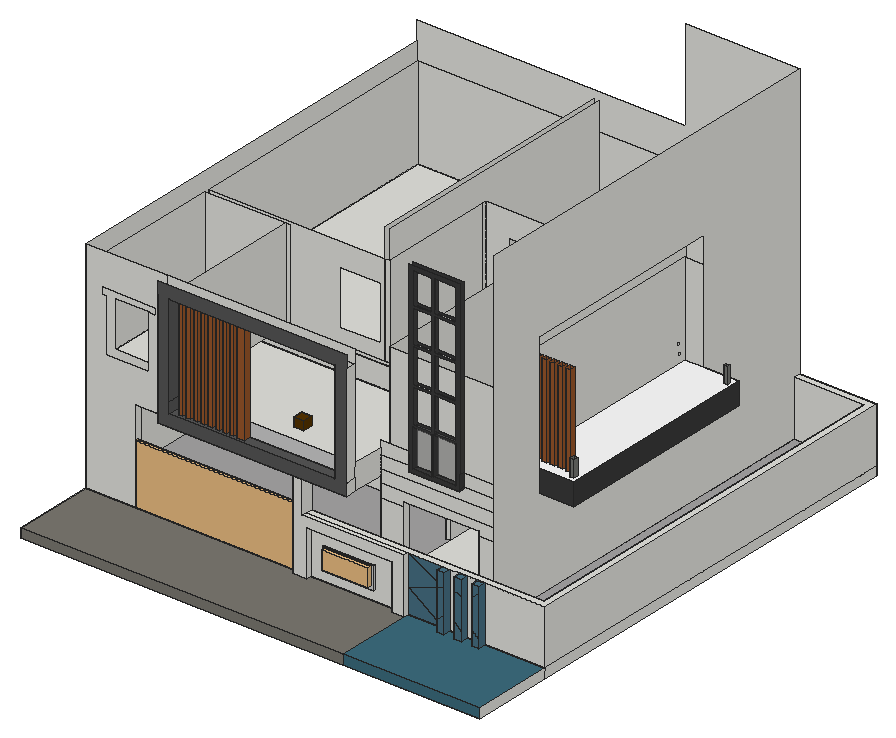
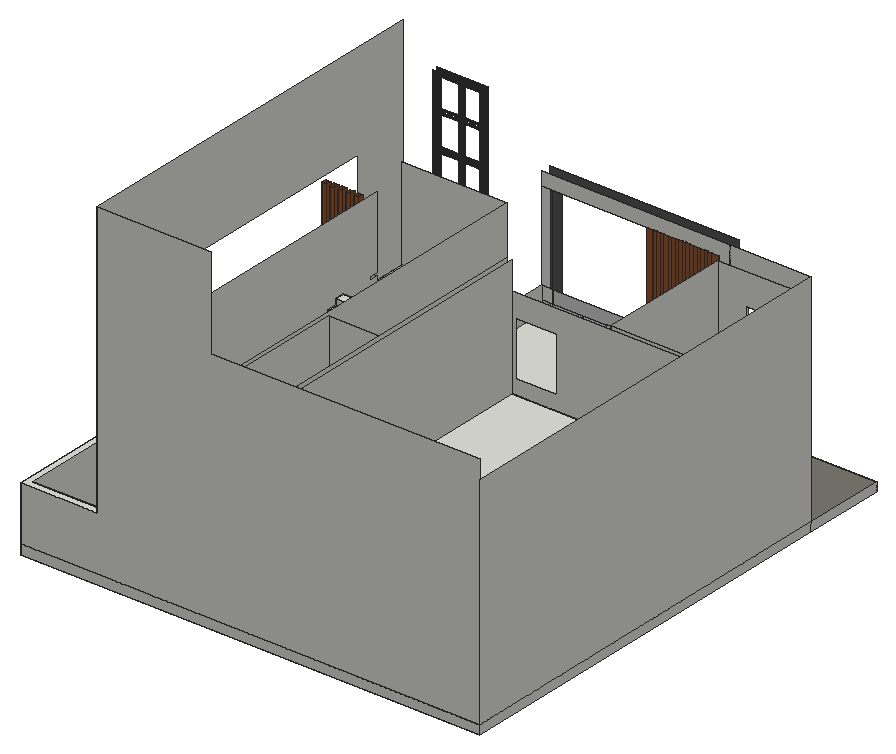
# SketchUp Ruby script. Lengths in inches.
U = 1.inch
M = Sketchup.active_model
def pt(a) = Geom::Point3d.new(a.map { |v| v * U })
def face(e, loops, mat)
  f = e.add_face(loops[0].map { |a| pt(a) })
  loops[1..].each { |l| e.add_face(l.map { |a| pt(a) }).erase! }
  f.material = f.back_material = mat if mat
  f
end
# faces: each face lists its corners as indices into pts; further lists are holes
def faces(e, pts, list, mat = nil) = list.each { |f| face(e, (f[0].is_a?(Array) ? f : [f]).map { |l| l.map { |i| pts[i] } }, mat) }
# xy, xz, yz: faces in a plane at the given z, y or x. An outline is a flat list of corners, or four numbers for a rectangle; further outlines are holes
def ring(l) = l.size == 4 ? [[l[0], l[1]], [l[2], l[1]], [l[2], l[3]], [l[0], l[3]]] : l.each_slice(2).to_a
def flat(e, list, mat, &to3) = list.each { |f| face(e, (f[0].is_a?(Array) ? f : [f]).map { |l| ring(l).map { |u, v| to3.(u, v) } }, mat) }
def xy(e, z, list, mat = nil) = flat(e, list, mat) { |x, y| [x, y, z] }
def xz(e, y, list, mat = nil) = flat(e, list, mat) { |x, z| [x, y, z] }
def yz(e, x, list, mat = nil) = flat(e, list, mat) { |y, z| [x, y, z] }
def lines(e, pts, list) = list.each { |a, b| e.add_line(pt(pts[a]), pt(pts[b])) }
# prism: a flat outline (further loops are holes) pulled along v
def prism(e, loops, v, mat = nil)
  f = face(e, loops, mat); d = Geom::Vector3d.new(v.map { |x| x * U })
  f.pushpull(f.normal.samedirection?(d) ? d.length : -d.length)
end
def box(e, o, s, mat = nil) = prism(e, [[o, [o[0] + s[0], o[1], o[2]], [o[0] + s[0], o[1] + s[1], o[2]], [o[0], o[1] + s[1], o[2]]]], [0, 0, s[2]], mat)
def at(x, y, z, deg = 0) = Geom::Transformation.translation(pt([x, y, z])) * Geom::Transformation.rotation(ORIGIN, Z_AXIS, deg.degrees)
def axes(o, x, y, z) = Geom::Transformation.new([*x, 0, *y, 0, *z, 0, *pt(o).to_a, 1])
def part(name) = M.definitions.add(name)
# library, detail: a bought-in or finely detailed component or shape, given as its bounding box
def library(name, o, s) = part(name).tap { |d| box(d.entities, o, s) }
def detail(e, o, s) = box(e.add_group.entities, o, s)
def put(e, d, t, mat = nil) = e.add_instance(d, t).tap { |i| i.material = mat if mat }
def group(e, t, mat = nil) = e.add_group.tap { |g| g.transformation = t; g.material = mat if mat }.entities
root = M.entities
M.materials.add("[Carrera Marble]").color = [207, 207, 207]
M.materials.add("[Color B08]").color = [63, 25, 0]
M.materials.add("[Color C05]").color = [255, 93, 0]
M.materials.add("[Color C08]").color = [74, 47, 0]
M.materials.add("[Color C08]1").color = [84, 51, 0]
M.materials.add("[Color M00]").color = [255, 255, 255]
M.materials.add("[Color M06]").color = [86, 86, 86]
M.materials.add("[Color M07]").color = [58, 58, 58]
M.materials.add("[Metal Seamed]").color = [118, 119, 115]
M.materials.add("[Rough Square Concrete Block]").color = [123, 120, 113]
M.materials.add("[Rough Square Concrete Block]1").color = [60, 108, 125]
M.materials.add("[Sketchy Lines Wavy Vertical]").color = [71, 112, 132]
M.materials.add("[Stone Vein Gray]").color = [166, 165, 165]
M.materials.add("[Translucent Glass Gray]").color = [128, 128, 128]
M.materials["[Translucent Glass Gray]"].alpha = 0.5
M.materials.add("[Wood Cherry Original]").color = [152, 86, 42]
c1 = part("Group\#3")
xy(c1.entities,0,[[0,0,48,8.5625]],"[Color C08]")
xy(c1.entities,4.98,[[4.98,0,43.02,2.5625],[4.98,2.5625,43.02,8.5625]],"[Color C08]")
xy(c1.entities,79.02,[[4.98,0,43.02,2.5625],[4.98,2.5625,43.02,8.5625]],"[Color C08]")
xy(c1.entities,84,[[0,0,48,8.5625]],"[Color C08]")
xz(c1.entities,0,[[[0,0,48,84],[4.98,4.98,43.02,79.02]]],"[Color C08]")
xz(c1.entities,2.5625,[[4.98,4.98,43.02,79.02]],"[Color C05]")
xz(c1.entities,8.5625,[[[0,0,48,84],[4.98,4.98,43.02,79.02]]],"[Color C08]")
yz(c1.entities,0,[[0,0,8.5625,84]],"[Color C08]")
yz(c1.entities,4.98,[[0,4.98,2.5625,79.02],[2.5625,4.98,8.5625,79.02]],"[Color C08]")
yz(c1.entities,43.02,[[0,4.98,2.5625,79.02],[2.5625,4.98,8.5625,79.02]],"[Color C08]")
yz(c1.entities,48,[[0,0,8.5625,84]],"[Color C08]")
c2 = library("Group\#6",[0,0,0],[195.5625,6,157.375])
c3 = library("RAMA",[0.59,0,0],[102.88,23.44,4])
c4 = library("Group\#4",[0,0,0],[48,6,60])
xy(root,0,[[0,0,600,106.4375],[0,106.4375,600,646.4375]])
xy(root,12,[[466.06,96.75,475.78,106.4375],[488.49,96.75,498.22,106.4375],[511.87,96.75,521.6,106.4375],[275.25,100.25,293.82,106.4375],[404.82,100.25,420.43,106.4375],
  [0,106.4375,0,646.4375,500,646.4375,500,147.79,480.58,147.79,480.58,155.92,494,155.92,494,637.4375,358,637.4375,358,254.07,352,254.07,352,290.0625,310.71,290.0625,310.71,296.0625,352,296.0625,352,637.4375,9,637.4375,9,296.0625,262.71,296.0625,262.71,290.0625,9,290.0625,9,115.4375,65.5625,115.4375,65.5625,106.4375],[65.5625,106.4375,275.25,115.4375],[275.25,106.4375,591,115.4375],[591,106.4375,591,637.4375,500,637.4375,500,646.4375,600,646.4375,600,106.4375],[352,147.79,352,181.82,358,181.82,358,155.92,382.83,155.92,382.83,147.79],
  [382.83,147.79,480.58,155.92],[358,155.92,494,637.4375],[9,296.0625,352,637.4375]])
xy(root,12,[[219.05,172.4,231.92,185.27]],"[Color C08]1")
xy(root,12,[[0,0,420.43,0,420.43,100.25,404.82,100.25,404.82,106.4375,293.82,106.4375,293.82,100.25,275.25,100.25,275.25,106.4375,0,106.4375]],"[Rough Square Concrete Block]")
xy(root,12,[[420.43,0,600,0,600,106.4375,521.6,106.4375,521.6,96.75,511.87,96.75,511.87,106.4375,498.22,106.4375,498.22,96.75,488.49,96.75,488.49,106.4375,475.78,106.4375,475.78,96.75,466.06,96.75,466.06,106.4375,420.43,106.4375]],"[Rough Square Concrete Block]1")
xy(root,12,[[[9,115.4375,591,115.4375,591,637.4375,500,637.4375,500,147.79,352,147.79,352,181.82,358,181.82,358,254.07,352,254.07,352,290.0625,310.71,290.0625,310.71,296.0625,262.71,296.0625,262.71,290.0625,9,290.0625],[219.05,172.4,231.92,185.27]]],"[Stone Vein Gray]")
xy(root,25.76,[[311.96,104.25,377.46,106.4375]],"[Carrera Marble]")
xy(root,30.26,[[181.25,290.0625,236,296.0625]])
xy(root,54.51,[[311.96,104.25,377.46,106.4375]],"[Carrera Marble]")
xy(root,71,[[293.82,100.25,404.82,106.4375]])
xy(root,78.48,[[35.34,290.0625,64.46,296.0625]])
xy(root,84,[[287.57,100.25,420.43,106.4375],[287.57,106.4375,600,106.4375,600,646.4375,500,646.4375,500,637.4375,591,637.4375,591,115.4375,287.57,115.4375]])
xy(root,84,[[466.06,96.75,475.78,106.4375],[488.49,96.75,498.22,106.4375],[511.87,96.75,521.6,106.4375]],"[Sketchy Lines Wavy Vertical]")
xy(root,96,[[262.71,290.0625,310.71,296.0625]])
xy(root,98.19,[[181.25,290.0625,236,296.0625]])
xy(root,107.99,[[352,181.82,358,254.07]])
xy(root,110.54,[[35.34,290.0625,64.46,296.0625]])
xy(root,112.31,[[382.83,147.79,480.58,155.92]])
xy(root,132,[[105.8,92.4375,105.8,106.4375,275.25,106.4375,275.25,100.25,287.57,100.25,287.57,106.4375,352,106.4375,352,92.4375],[275.25,100.25,287.57,106.4375],[65.5625,106.4375,65.5625,115.4375,9,115.4375,9,290.0625,352,290.0625,352,106.4375,287.57,106.4375,287.57,115.4375,275.25,115.4375,275.25,106.4375],[275.25,106.4375,287.57,115.4375]])
xy(root,132,[[500,220.28,546,489.49]],"[Color M07]")
xy(root,143.25,[[219.05,172.4,231.92,185.27]],"[Color C08]1")
xy(root,147.1875,[[120,92.4375,336.97,92.4375,336.97,106.4375,214.79,106.4375,214.79,96.98,205.34,96.98,205.34,106.4375,201.17,106.4375,201.17,97.4375,195.61,97.4375,195.61,106.4375,191.67,106.4375,191.67,97.4375,186.11,97.4375,186.11,106.4375,182.17,106.4375,182.17,97.4375,176.61,97.4375,176.61,106.4375,172.67,106.4375,172.67,97.4375,167.11,97.4375,167.11,106.4375,163.17,106.4375,163.17,97.4375,157.61,97.4375,157.61,106.4375,153.67,106.4375,153.67,97.4375,148.11,97.4375,148.11,106.4375,144.17,106.4375,144.17,97.4375,138.61,97.4375,138.61,106.4375,134.67,106.4375,134.67,97.4375,129.11,97.4375,129.11,106.4375,120,106.4375]],"[Color M06]")
xy(root,147.1875,[[205.34,96.98,214.79,106.4375],[129.11,97.4375,134.67,106.4375],[138.61,97.4375,144.17,106.4375],[148.11,97.4375,153.67,106.4375],[157.61,97.4375,163.17,106.4375],
  [167.11,97.4375,172.67,106.4375],[176.61,97.4375,182.17,106.4375],[186.11,97.4375,191.67,106.4375],[195.61,97.4375,201.17,106.4375]],"[Wood Cherry Original]")
xy(root,154.54,[[394.33,141.23,460.92,147.79]],"[Color M07]")
xy(root,157,[[9,296.0625,352,637.4375]])
xy(root,159.46,[[399.25,141.23,424.3125,147.79],[427.08,141.23,456,147.79]],"[Color M07]")
xy(root,161,[[9,115.4375,114,290.0625],[9,296.0625,238.75,637.4375],[238.75,296.0625,244.75,637.4375],[244.75,296.0625,286.54,453.4375],[286.54,296.0625,352,453.4375],
  [244.75,453.4375,352,637.4375]])
xy(root,161,[[[475.4375,220.28,546,489.49],[525.05,234.2,531.37,240.63],[514.62,234.2,520.93,240.63],[503.93,234.2,510.24,240.63],[482.87,234.2,489.18,240.63],[493.55,234.2,499.87,240.57],[536.02,226.32,541.65,232.26],[536.58,476.42,541.89,480.67]]],"[Color M00]")
xy(root,161,[[536.02,226.32,541.65,232.26],[536.58,476.42,541.89,480.67]],"[Metal Seamed]")
xy(root,161,[[482.87,234.2,489.18,240.63],[503.93,234.2,510.24,240.63],[514.62,234.2,520.93,240.63],[525.05,234.2,531.37,240.63]],"[Wood Cherry Original]")
xz(root,0,[[0,0,420.43,12]],"[Rough Square Concrete Block]")
xz(root,0,[[420.43,0,600,12]],"[Rough Square Concrete Block]1")
xz(root,92.4375,[[[105.8,132,352,298],[120,147.1875,336.97,281]]],"[Color M06]")
xz(root,96.75,[[466.06,12,475.78,12,475.78,34.11,466.06,26.11],[488.49,12,498.22,12,498.22,22.65,488.49,34.11],[511.87,12,521.6,12,521.6,22.65,511.87,29.1875],[498.22,22.65,498.22,63.7,488.49,68.19,488.49,34.11],[521.6,22.65,521.6,75.375,511.87,68.19,511.87,29.1875],
  [466.06,26.11,475.78,34.11,475.78,68.19,466.06,63.7],[466.06,63.7,475.78,68.19,475.78,84,466.06,84],[498.22,63.7,498.22,84,488.49,84,488.49,68.19],[511.87,68.19,521.6,75.375,521.6,84,511.87,84]],"[Sketchy Lines Wavy Vertical]")
xz(root,96.98,[[205.34,147.1875,214.79,281]],"[Wood Cherry Original]")
xz(root,97.4375,[[129.11,147.1875,134.67,281],[138.61,147.1875,144.17,281],[148.11,147.1875,153.67,281],[157.61,147.1875,163.17,281.25],[167.11,147.1875,172.67,281.125],
  [176.61,147.1875,182.17,281],[186.11,147.1875,191.67,280.8125],[195.61,147.1875,201.17,281]],"[Wood Cherry Original]")
xz(root,100.25,[[275.25,12,293.82,12,293.82,71,404.82,71,404.82,12,420.43,12,420.43,84,287.57,84,287.57,132,275.25,132]])
xz(root,104.25,[[311.96,25.76,377.46,54.51]],"[Carrera Marble]")
xz(root,106.4375,[[0,0,600,12],[[0,12,65.5625,12,65.5625,132,105.8,132,105.8,298,0,298],[25.93,176.87,25.93,245.68,20.68,245.68,20.68,255.3,92.11,255.3,92.11,245.68,82.74,245.68,82.74,176.87]],[[293.82,12,404.82,71],[311.96,25.76,377.46,54.51]],[466.06,12,475.78,84],[475.78,12,488.49,84],
  [488.49,12,498.22,84],[498.22,12,511.87,84],[511.87,12,521.6,84],[521.6,12,600,84],[105.8,132,105.8,298,352,298,352,281,172.67,281,172.67,281.125,167.11,281.125,167.11,281,163.17,281,163.17,281.25,157.61,281.25,157.61,281,120,281,120,147.1875,352,147.1875,352,132],
  [336.97,147.1875,352,164.875]])
xz(root,106.4375,[[214.79,147.1875,336.97,164.875]],"[Carrera Marble]")
xz(root,106.4375,[[120,147.1875,129.11,164.875],[129.11,147.1875,134.67,164.875],[134.67,147.1875,138.61,164.875],[138.61,147.1875,144.17,164.875],[144.17,147.1875,148.11,164.875],
  [148.11,147.1875,153.67,164.875],[153.67,147.1875,157.61,164.875],[157.61,147.1875,163.17,164.875],[163.17,147.1875,167.11,164.875],[167.11,147.1875,172.67,164.875],
  [172.67,147.1875,176.61,164.875],[176.61,147.1875,182.17,164.875],[182.17,147.1875,186.11,164.875],[186.11,147.1875,191.67,164.875],[191.67,147.1875,195.61,164.875],
  [195.61,147.1875,201.17,164.875],[201.17,147.1875,205.34,164.875],[205.34,147.1875,214.79,164.875]],"[Color M06]")
xz(root,106.4375,[[420.43,12,466.06,12,420.43,43.83],[466.06,12,466.06,59.11,420.43,43.83],[420.43,43.83,466.06,59.11,420.43,84],[466.06,59.11,466.06,84,420.43,84]],"[Sketchy Lines Wavy Vertical]")
xz(root,115.4375,[[9,12,65.5625,132],[275.25,12,275.25,132,287.57,132,287.57,84,591,84,591,12],[[9,161,114,281],[30.34,181.27,78.34,241.27]]])
xz(root,141.23,[[[394.33,154.54,460.92,397.01],[427.08,159.46,456,208.53],[427.08,257.48,456,302.9],[427.08,210.6,456,255.4],[427.08,304.98,456,348.22],[399.25,159.46,424.3125,208.53],[427.08,350.29,456,392.08],[399.25,257.48,424.3125,302.9],[399.25,210.6,424.3125,255.4],[399.25,304.98,424.3125,348.22],[399.25,350.29,424.3125,392.08]]],"[Color M07]")
xz(root,147.79,[[352,12,382.83,106.6],[480.58,12,500,106.6],[352,106.6,382.83,106.6,382.83,112.31,480.58,112.31,480.58,106.6,500,106.6,500,123.35,352,123.35],[352,123.35,500,140.1],[352,140.1,500,140.1,500,156.85,460.92,156.85,460.92,154.54,394.33,154.54,394.33,156.85,352,156.85],
  [352,156.85,394.33,173.6],[460.92,156.85,500,173.6]])
xz(root,147.79,[[[394.33,154.54,460.92,397.01],[427.08,159.46,456,208.53],[427.08,257.48,456,302.9],[427.08,210.6,456,255.4],[427.08,304.98,456,348.22],[399.25,159.46,424.3125,208.53],[427.08,350.29,456,392.08],[399.25,257.48,424.3125,302.9],[399.25,210.6,424.3125,255.4],[399.25,304.98,424.3125,348.22],[399.25,350.29,424.3125,392.08]]],"[Color M07]")
xz(root,147.79,[[399.25,159.46,424.3125,208.53],[427.08,159.46,456,208.53]],"[Translucent Glass Gray]")
xz(root,155.92,[[358,12,358,281,494,281,494,12,480.58,12,480.58,112.31,382.83,112.31,382.83,12]])
xz(root,172.4,[[219.05,12,231.92,143.25]],"[Color C08]1")
xz(root,181.82,[[352,12,358,107.99]])
xz(root,185.27,[[219.05,12,231.92,143.25]],"[Color C08]1")
xz(root,220.28,[[475.4375,161,500,181.87]])
xz(root,220.28,[[500,132,546,161]],"[Color M07]")
xz(root,226.32,[[536.02,161,541.65,182.4375]],"[Metal Seamed]")
xz(root,232.26,[[536.02,161,541.65,182.4375]],"[Metal Seamed]")
xz(root,234.2,[[482.87,161,489.18,281],[493.55,161,499.87,281],[503.93,161,510.24,281],[514.62,161,520.93,281],[525.05,161,531.37,281.1875]],"[Wood Cherry Original]")
xz(root,240.57,[[493.55,161,499.87,281]],"[Wood Cherry Original]")
xz(root,240.63,[[482.87,161,489.18,281],[503.93,161,510.24,281],[514.62,161,520.93,281],[525.05,161,531.37,281.1875]],"[Wood Cherry Original]")
xz(root,254.07,[[352,12,358,107.99]])
xz(root,290.0625,[[[9,12,262.71,12,262.71,96,310.71,96,310.71,12,352,12,352,132,9,132],[181.25,30.26,236,98.19],[35.34,78.48,64.46,110.54]],[9,132,352,161],[9,161,114,281],[114,161,120,281]])
xz(root,296.0625,[[[9,12,9,132,352,132,352,12,310.71,12,310.71,96,262.71,96,262.71,12],[181.25,30.26,236,98.19],[35.34,78.48,64.46,110.54]],[9,132,352,157],[9,157,286.54,161],[286.54,157,352,161],[[9,161,238.75,281],[180.25,179.95,233.4375,251.14]],
  [238.75,161,244.75,281]])
xz(root,453.4375,[[[244.75,161,352,281],[274.29,164.875,322.29,248.875]]])
xz(root,476.42,[[536.58,161,541.89,181.87]],"[Metal Seamed]")
xz(root,480.67,[[536.58,161,541.89,181.87]],"[Metal Seamed]")
xz(root,489.49,[[475.4375,161,500,281]])
xz(root,489.49,[[500,132,546,161]],"[Color M07]")
xz(root,637.4375,[[9,12,352,132],[358,12,494,132],[500,12,591,84],[9,132,352,157],[358,132,494,161],
  [9,157,352,161],[9,161,238.75,281],[238.75,161,244.75,281],[244.75,161,352,281],[358,161,494,281]])
xz(root,646.4375,[[0,0,600,12],[0,12,0,322,352,322,352,441.0625,500,441.0625,500,84,600,84,600,12]])
yz(root,0,[[0,0,106.4375,12],[106.4375,0,646.4375,12],[106.4375,12,646.4375,298]])
yz(root,9,[[115.4375,12,290.0625,132],[296.0625,12,637.4375,132],[115.4375,132,290.0625,161],[296.0625,132,637.4375,157],[296.0625,157,334.63,161],
  [334.63,157,356.32,161],[356.32,157,637.4375,161],[115.4375,161,290.0625,281],[296.0625,161,637.4375,281]])
yz(root,35.34,[[290.0625,78.48,296.0625,110.54]])
yz(root,64.46,[[290.0625,78.48,296.0625,110.54]])
yz(root,65.5625,[[106.4375,12,115.4375,132]])
yz(root,105.8,[[92.4375,132,106.4375,161],[92.4375,161,106.4375,281]])
yz(root,114,[[115.4375,161,290.0625,281]])
yz(root,120,[[92.4375,147.1875,106.4375,161],[92.4375,161,106.4375,281]],"[Color M06]")
yz(root,129.11,[[97.4375,147.1875,106.4375,281]],"[Wood Cherry Original]")
yz(root,134.67,[[97.4375,147.1875,106.4375,281]],"[Wood Cherry Original]")
yz(root,138.61,[[97.4375,147.1875,106.4375,281]],"[Wood Cherry Original]")
yz(root,144.17,[[97.4375,147.1875,106.4375,281]],"[Wood Cherry Original]")
yz(root,148.11,[[97.4375,147.1875,106.4375,281]],"[Wood Cherry Original]")
yz(root,153.67,[[97.4375,147.1875,106.4375,281]],"[Wood Cherry Original]")
yz(root,157.61,[[97.4375,147.1875,106.4375,281.25]],"[Wood Cherry Original]")
yz(root,163.17,[[97.4375,147.1875,106.4375,281.25]],"[Wood Cherry Original]")
yz(root,167.11,[[97.4375,147.1875,106.4375,281.125]],"[Wood Cherry Original]")
yz(root,172.67,[[97.4375,147.1875,106.4375,281.125]],"[Wood Cherry Original]")
yz(root,176.61,[[97.4375,147.1875,106.4375,281]],"[Wood Cherry Original]")
yz(root,181.25,[[290.0625,30.26,296.0625,98.19]])
yz(root,182.17,[[97.4375,147.1875,106.4375,281]],"[Wood Cherry Original]")
yz(root,186.11,[[97.4375,147.1875,106.4375,280.8125]],"[Wood Cherry Original]")
yz(root,191.67,[[97.4375,147.1875,106.4375,280.8125]],"[Wood Cherry Original]")
yz(root,195.61,[[97.4375,147.1875,106.4375,281]],"[Wood Cherry Original]")
yz(root,201.17,[[97.4375,147.1875,106.4375,281]],"[Wood Cherry Original]")
yz(root,205.34,[[96.98,147.1875,106.4375,281]],"[Wood Cherry Original]")
yz(root,214.79,[[96.98,147.1875,106.4375,281]],"[Wood Cherry Original]")
yz(root,219.05,[[172.4,12,185.27,143.25]],"[Color C08]1")
yz(root,231.92,[[172.4,12,185.27,143.25]],"[Color C08]1")
yz(root,236,[[290.0625,30.26,296.0625,98.19]])
yz(root,238.75,[[296.0625,161,637.4375,318]])
yz(root,244.75,[[296.0625,161,453.4375,161,453.4375,281,449.1875,281,449.1875,164.875,296.0625,164.875],[453.4375,161,637.4375,161,637.4375,318,296.0625,318,296.0625,281,453.4375,281]])
yz(root,262.71,[[290.0625,12,296.0625,96]])
yz(root,275.25,[[100.25,12,106.4375,132],[106.4375,12,115.4375,132]])
yz(root,287.57,[[100.25,84,115.4375,132]])
yz(root,293.82,[[100.25,12,106.4375,71]])
yz(root,310.71,[[290.0625,12,296.0625,96]])
yz(root,311.96,[[104.25,25.76,106.4375,54.51]],"[Carrera Marble]")
yz(root,336.97,[[92.4375,147.1875,106.4375,281]],"[Color M06]")
yz(root,352,[[147.79,12,147.79,132,290.0625,132,290.0625,12,254.07,12,254.07,107.99,181.82,107.99,181.82,12],[296.0625,12,637.4375,132],[92.4375,132,106.4375,147.1875],[106.4375,132,147.79,164.875],[147.79,132,290.0625,161],
  [296.0625,132,637.4375,157],[92.4375,147.1875,106.4375,281],[296.0625,157,637.4375,161],[147.79,161,290.0625,164.875],[453.4375,161,637.4375,281]])
yz(root,358,[[155.92,12,181.82,12,181.82,107.99,254.07,107.99,254.07,12,637.4375,12,637.4375,132,155.92,132],[155.92,132,637.4375,161],[155.92,161,637.4375,281]])
yz(root,377.46,[[104.25,25.76,106.4375,54.51]],"[Carrera Marble]")
yz(root,382.83,[[147.79,12,155.92,112.31]])
yz(root,394.33,[[141.23,154.54,147.79,156.85],[141.23,156.85,147.79,173.6]],"[Color M07]")
yz(root,399.25,[[141.23,159.46,147.79,208.53]],"[Color M07]")
yz(root,404.82,[[100.25,12,106.4375,71]])
yz(root,420.43,[[100.25,12,106.4375,84]])
yz(root,424.3125,[[141.23,159.46,147.79,208.53]],"[Color M07]")
yz(root,427.08,[[141.23,159.46,147.79,208.53]],"[Color M07]")
yz(root,456,[[141.23,159.46,147.79,208.53]],"[Color M07]")
yz(root,460.92,[[141.23,154.54,147.79,156.85],[141.23,156.85,147.79,173.6]],"[Color M07]")
yz(root,466.06,[[96.75,12,106.4375,84]],"[Sketchy Lines Wavy Vertical]")
yz(root,475.4375,[[[220.28,161,489.49,161,489.49,281,220.28,281,220.28,186.3125,231.31,186.3125,231.31,181.87,220.28,181.87],[476.33,181.87,481.18,186.3125],[478.41,169.04,483.17,173.48],[224.05,169.04,228.48,173.48]]])
yz(root,475.78,[[96.75,12,106.4375,84]],"[Sketchy Lines Wavy Vertical]")
yz(root,480.58,[[147.79,12,155.92,112.31]])
yz(root,482.87,[[234.2,161,240.63,281]],"[Wood Cherry Original]")
yz(root,488.49,[[96.75,12,106.4375,84]],"[Sketchy Lines Wavy Vertical]")
yz(root,489.18,[[234.2,161,240.63,281]],"[Wood Cherry Original]")
yz(root,493.55,[[234.2,161,240.57,281]],"[Wood Cherry Original]")
yz(root,494,[[155.92,12,637.4375,132]])
yz(root,498.22,[[96.75,12,106.4375,84]],"[Sketchy Lines Wavy Vertical]")
yz(root,499.87,[[234.2,161,240.57,281]],"[Wood Cherry Original]")
yz(root,500,[[[147.79,12,637.4375,12,637.4375,84,646.4375,84,646.4375,441.0625,147.79,441.0625],[220.28,132,489.49,315]]])
yz(root,503.93,[[234.2,161,240.63,281]],"[Wood Cherry Original]")
yz(root,510.24,[[234.2,161,240.63,281]],"[Wood Cherry Original]")
yz(root,511.87,[[96.75,12,106.4375,84]],"[Sketchy Lines Wavy Vertical]")
yz(root,514.62,[[234.2,161,240.63,281]],"[Wood Cherry Original]")
yz(root,520.93,[[234.2,161,240.63,281]],"[Wood Cherry Original]")
yz(root,521.6,[[96.75,12,106.4375,84]],"[Sketchy Lines Wavy Vertical]")
yz(root,525.05,[[234.2,161,240.63,281.1875]],"[Wood Cherry Original]")
yz(root,531.37,[[234.2,161,240.63,281.1875]],"[Wood Cherry Original]")
yz(root,536.02,[[226.32,161,232.26,182.4375]],"[Metal Seamed]")
yz(root,536.58,[[476.42,161,480.67,181.87]],"[Metal Seamed]")
yz(root,541.65,[[226.32,161,232.26,182.4375]],"[Metal Seamed]")
yz(root,541.89,[[476.42,161,480.67,181.87]],"[Metal Seamed]")
yz(root,546,[[220.28,132,489.49,161]],"[Color M07]")
yz(root,591,[[115.4375,12,637.4375,84]])
yz(root,600,[[0,0,106.4375,12],[106.4375,0,646.4375,12],[106.4375,12,646.4375,84]])
p = [[494,155.92,161],[494,220.28,161],[114,106.4375,161],[114,115.4375,161],[286.54,296.0625,161],[261.27,293.0625,161],
  [236,290.0625,161],[494,489.49,161],[494,637.4375,161]]
lines(root,p,[[0,1],[2,3],[4,5],[5,6],[7,8]])
g1 = group(root,at(365.21,290.34,12))
xy(g1,0,[[0,0,50.3125,12],[0,12,50.3125,126.625],[0,126.625,50.3125,132]])
xy(g1,8,[[0,0,50.3125,12]])
xy(g1,16,[[0,12,50.3125,24]])
xy(g1,24,[[0,24,50.3125,36]])
xy(g1,32,[[0,36,50.3125,48]])
xy(g1,40,[[0,48,50.3125,60]])
xy(g1,48,[[0,60,50.3125,72]])
xy(g1,56,[[0,72,50.3125,84]])
xy(g1,64,[[0,84,50.3125,96]])
xy(g1,72,[[0,96,50.3125,108]])
xy(g1,80,[[0,108,50.3125,120]])
xy(g1,88,[[0,120,50.3125,132],[0,132,98.0625,166.5625]])
xy(g1,96,[[0,132,98.0625,166.5625]])
xz(g1,0,[[0,0,50.3125,8]])
xz(g1,12,[[0,8,50.3125,16]])
xz(g1,24,[[0,16,50.3125,24]])
xz(g1,36,[[0,24,50.3125,32]])
xz(g1,48,[[0,32,50.3125,40]])
xz(g1,60,[[0,40,50.3125,48]])
xz(g1,72,[[0,48,50.3125,56]])
xz(g1,84,[[0,56,50.3125,64]])
xz(g1,96,[[0,64,50.3125,72]])
xz(g1,108,[[0,72,50.3125,80]])
xz(g1,120,[[0,80,50.3125,88]])
xz(g1,132,[[0,0,50.3125,80],[0,80,50.3125,88],[0,88,98.0625,96]])
xz(g1,166.5625,[[0,88,98.0625,96]])
yz(g1,0,[[0,0,0,8,12,8,12,16,24,16,24,24,36,24,36,32,48,32,48,40,60,40,60,48,72,48,72,56,84,56,84,64,96,64,96,72,108,72,108,80,120,80,120,88,132,88,132,0],[132,88,166.5625,96]])
yz(g1,50.3125,[[0,0,132,0,132,88,120,88,120,80,108,80,108,72,96,72,96,64,84,64,84,56,72,56,72,48,60,48,60,40,48,40,48,32,36,32,36,24,24,24,24,16,12,16,12,8,0,8]])
yz(g1,98.0625,[[132,88,166.5625,96]])
g2 = group(g1,at(48.3125,0,96))
prism(g2,[[[50.3125,36,72],[50.3125,24,72],[50.3125,24,80],[50.3125,12,80],[50.3125,12,88],[50.3125,0,88],[50.3125,0,3.125],[50.3125,120,0],[50.3125,132,0],[50.3125,132,8],[50.3125,120,8],[50.3125,120,16],[50.3125,108,16],[50.3125,108,24],[50.3125,96,24],[50.3125,96,32],[50.3125,84,32],[50.3125,84,40],[50.3125,72,40],[50.3125,72,48],[50.3125,60,48],[50.3125,60,56],[50.3125,48,56],[50.3125,48,64],[50.3125,36,64]]],[-50.3125,0,0])
put(root,c1,at(262.71,290.0625,12))
put(root,c2,axes([65.5625,106.4375,12],[1.07221,0,0],[0,0.5,0],[0,0,0.5]))
put(root,c3,axes([313.4,104.25,29.61],[0.58154,0,0],[0,0,1],[0,-1,0]),"[Color M06]")
put(root,c4,axes([181.25,290.0625,30.26],[1.14062,0,0],[0,1,0],[0,0,1.13229]))
g3 = group(root,at(35.34,290.0625,78.48))
xy(g3,0,[[0,0,29.125,6]],"[Color B08]")
xy(g3,3.05,[[2.77,0,26.36,6]],"[Color B08]")
xy(g3,29.01,[[2.77,0,26.36,6]],"[Color B08]")
xy(g3,32.0625,[[0,0,29.125,6]],"[Color B08]")
xz(g3,0,[[[0,0,29.125,32.0625],[2.77,3.05,26.36,29.01]]],"[Color B08]")
xz(g3,0,[[2.77,3.05,26.36,29.01]],"[Translucent Glass Gray]")
xz(g3,6,[[[0,0,29.125,32.0625],[2.77,3.05,26.36,29.01]]],"[Color B08]")
yz(g3,0,[[0,0,6,32.0625]],"[Color B08]")
yz(g3,2.77,[[0,3.05,6,29.01]],"[Color B08]")
yz(g3,26.36,[[0,3.05,6,29.01]],"[Color B08]")
yz(g3,29.125,[[0,0,6,32.0625]],"[Color B08]")
